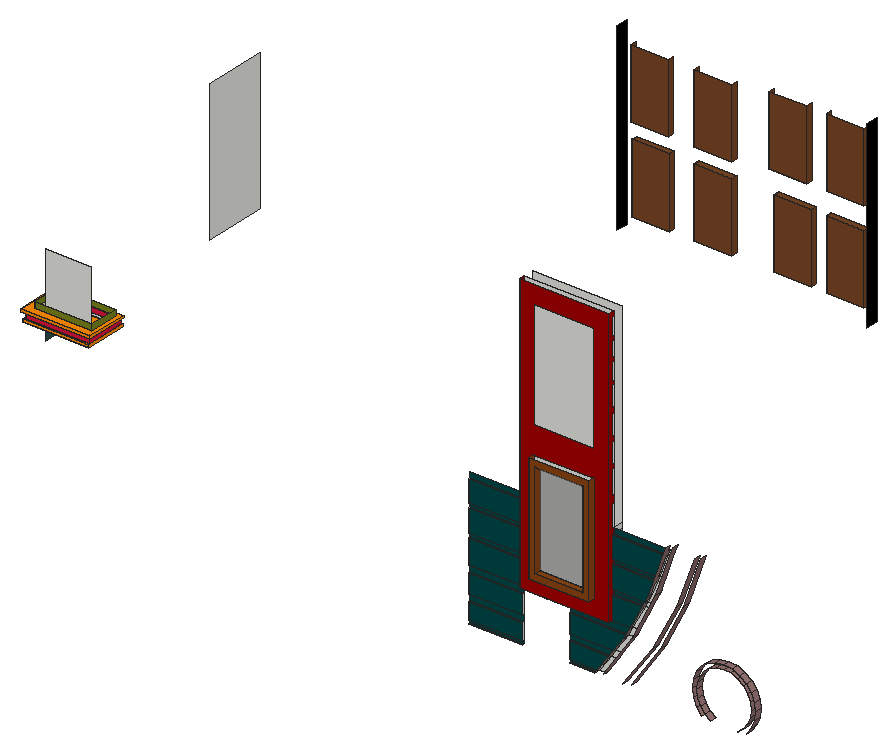
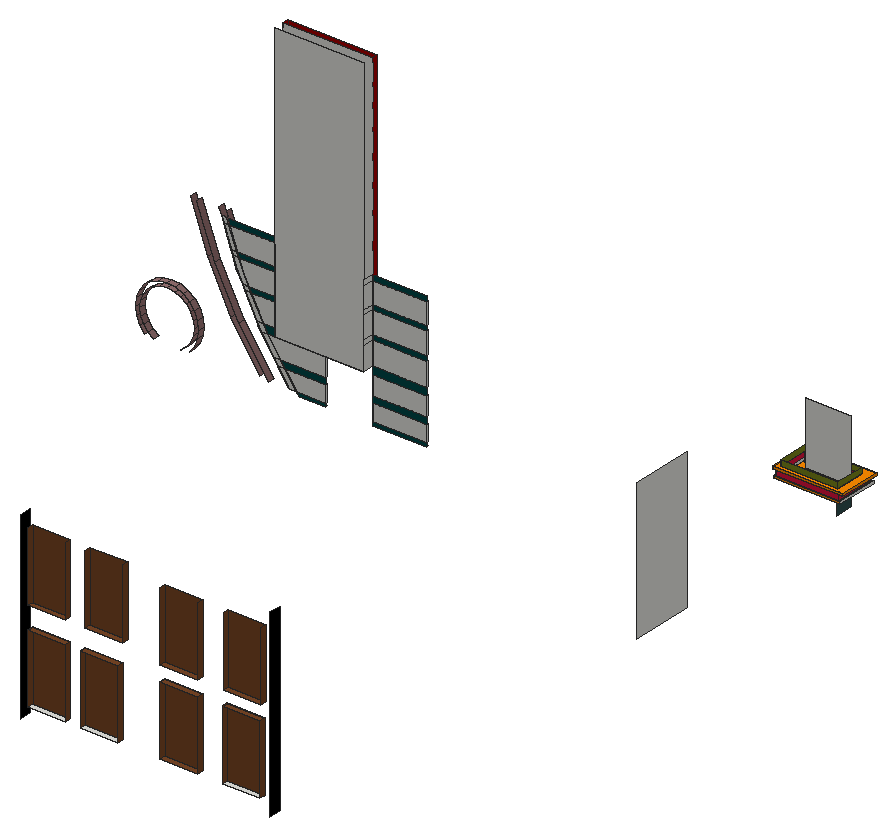
# SketchUp Ruby script. Lengths in inches.
U = 1.inch
M = Sketchup.active_model
def pt(a) = Geom::Point3d.new(a.map { |v| v * U })
def face(e, loops, mat)
  f = e.add_face(loops[0].map { |a| pt(a) })
  loops[1..].each { |l| e.add_face(l.map { |a| pt(a) }).erase! }
  f.material = f.back_material = mat if mat
  f
end
# faces: each face lists its corners as indices into pts; further lists are holes
def faces(e, pts, list, mat = nil) = list.each { |f| face(e, (f[0].is_a?(Array) ? f : [f]).map { |l| l.map { |i| pts[i] } }, mat) }
# xy, xz, yz: faces in a plane at the given z, y or x. An outline is a flat list of corners, or four numbers for a rectangle; further outlines are holes
def ring(l) = l.size == 4 ? [[l[0], l[1]], [l[2], l[1]], [l[2], l[3]], [l[0], l[3]]] : l.each_slice(2).to_a
def flat(e, list, mat, &to3) = list.each { |f| face(e, (f[0].is_a?(Array) ? f : [f]).map { |l| ring(l).map { |u, v| to3.(u, v) } }, mat) }
def xy(e, z, list, mat = nil) = flat(e, list, mat) { |x, y| [x, y, z] }
def xz(e, y, list, mat = nil) = flat(e, list, mat) { |x, z| [x, y, z] }
def yz(e, x, list, mat = nil) = flat(e, list, mat) { |y, z| [x, y, z] }
def lines(e, pts, list) = list.each { |a, b| e.add_line(pt(pts[a]), pt(pts[b])) }
# prism: a flat outline (further loops are holes) pulled along v
def prism(e, loops, v, mat = nil)
  f = face(e, loops, mat); d = Geom::Vector3d.new(v.map { |x| x * U })
  f.pushpull(f.normal.samedirection?(d) ? d.length : -d.length)
end
def box(e, o, s, mat = nil) = prism(e, [[o, [o[0] + s[0], o[1], o[2]], [o[0] + s[0], o[1] + s[1], o[2]], [o[0], o[1] + s[1], o[2]]]], [0, 0, s[2]], mat)
def at(x, y, z, deg = 0) = Geom::Transformation.translation(pt([x, y, z])) * Geom::Transformation.rotation(ORIGIN, Z_AXIS, deg.degrees)
def axes(o, x, y, z) = Geom::Transformation.new([*x, 0, *y, 0, *z, 0, *pt(o).to_a, 1])
def part(name) = M.definitions.add(name)
# library, detail: a bought-in or finely detailed component or shape, given as its bounding box
def library(name, o, s) = part(name).tap { |d| box(d.entities, o, s) }
def detail(e, o, s) = box(e.add_group.entities, o, s)
def put(e, d, t, mat = nil) = e.add_instance(d, t).tap { |i| i.material = mat if mat }
def group(e, t, mat = nil) = e.add_group.tap { |g| g.transformation = t; g.material = mat if mat }.entities
root = M.entities
M.materials.add("[0019_Crimson]").color = [220, 20, 60]
M.materials.add("[0020_Red]").color = [165, 0, 0]
M.materials.add("[0039_DarkOrange]").color = [255, 140, 0]
M.materials.add("[0043_SaddleBrown]").color = [139, 69, 19]
M.materials.add("[0057_DarkKhaki]").color = [122, 132, 27]
M.materials.add("[0078_DarkSlateGray]").color = [47, 79, 79]
M.materials.add("[0119_RosyBrown]").color = [150, 114, 114]
M.materials.add("[0137_Black]").color = [0, 0, 0]
M.materials.add("[Color H08]").color = [0, 71, 71]
M.materials.add("[Translucent Glass Gray]").color = [128, 128, 128]
M.materials["[Translucent Glass Gray]"].alpha = 0.5
M.materials.add("[Wood Veneer 01]").color = [120, 70, 37]
xy(root,126.49,[[221.0625,650.11,247.97,651.11],[271.25,650.11,284.14,651.11]],"[Color H08]")
xy(root,128.2,[[221.0625,650.11,247.97,651.11],[271.25,650.11,285.64,651.11]],"[Color H08]")
xy(root,136.45,[[221.0625,650.11,247.97,651.11],[271.25,650.11,291.42,651.11]],"[Color H08]")
xy(root,139.3125,[[82.93,924.36,101.74,927.36],[153.68,924.36,172.49,927.36],[179.93,924.36,198.74,927.36]])
xy(root,139.3125,[[114.12,924.36,132.93,927.36]],"[Wood Veneer 01]")
xy(root,139.72,[[221.0625,650.11,247.97,651.11],[271.25,650.11,293.72,651.11]],"[Color H08]")
xy(root,149.04,[[221.0625,650.11,247.97,651.11],[271.25,650.11,300.25,651.11]],"[Color H08]")
xy(root,152.96,[[252.74,648.11,252.74,649.11,247.97,649.11,247.97,651.11,271.25,651.11,271.25,649.11,266.58,649.11,266.58,648.11,265.61,648.11,265.61,649.11,253.7,649.11,253.7,648.11],[257.51,648.11,259.2,649.11],[261.76,648.11,263.45,649.11],[247.97,651.11,292.45,656.36]])
xy(root,152.96,[[247.97,648.11,252.74,649.11],[253.7,648.11,257.51,649.11],[259.2,648.11,261.76,649.11],[263.45,648.11,265.61,649.11],[266.58,648.11,266.58,649.11,271.25,649.11,271.25,651.11,292.45,651.11,292.45,648.11]],"[0020_Red]")
xy(root,152.96,[[221.0625,650.11,247.97,651.11],[292.45,650.11,302.3,651.11]],"[Color H08]")
xy(root,160.75,[[255.01,645.11,284.88,648.11]],"[0043_SaddleBrown]")
xy(root,163.75,[[258.01,645.11,281.88,648.11]],"[0043_SaddleBrown]")
xy(root,164.61,[[221.0625,650.11,247.97,651.11],[292.45,650.11,308.39,651.11]],"[Color H08]")
xy(root,166.89,[[221.0625,650.11,247.97,651.11],[292.45,650.11,309.58,651.11]],"[Color H08]")
xy(root,173.8125,[[82.93,924.36,101.74,927.36],[114.12,924.36,132.93,927.36],[153.68,924.36,172.49,927.36],[179.93,924.36,198.74,927.36]],"[Wood Veneer 01]")
xy(root,178.2,[[221.0625,650.11,247.97,651.11],[292.45,650.11,314.52,651.11]],"[Color H08]")
xy(root,180.47,[[221.0625,650.11,247.97,651.11],[292.45,650.11,315.35,651.11]],"[Color H08]")
xy(root,181.25,[[82.37,924.36,101.18,927.36],[114.12,924.36,132.93,927.36]],"[Wood Veneer 01]")
xy(root,184.8125,[[151.49,924.36,170.3,927.36],[179.93,924.36,198.74,927.36]],"[Wood Veneer 01]")
xy(root,185.51,[[7,654.11,29.57,663.11]])
xy(root,185.52,[[2.1875,648.11,33.82,667.68]],"[0039_DarkOrange]")
xy(root,185.54,[[[1.375,647.11,34.38,668.24],[2.1875,648.11,33.82,667.68]]],"[0039_DarkOrange]")
xy(root,186.71,[[33.82,667.68,34.38,668.24]])
xy(root,186.71,[[1.375,647.11,34.38,647.11,34.38,667.68,33.82,667.68,33.82,648.11,2.1875,648.11,2.1875,667.68,33.82,667.68,33.82,668.24,1.375,668.24]],"[0039_DarkOrange]")
xy(root,189.54,[[0,647.11,0,667.68,2.1875,667.68,2.1875,648.11,34.75,648.11,34.75,647.11],[33.82,648.11,33.82,667.68,0,667.68,0,668.24,34.75,668.24,34.75,648.11]],"[0039_DarkOrange]")
xy(root,190.71,[[[0,647.11,34.75,668.24],[4,651.11,32.57,666.11]]],"[0039_DarkOrange]")
xy(root,191.16,[[221.0625,650.11,247.97,651.11],[292.45,650.11,319.27,651.11]],"[Color H08]")
xz(root,645.11,[[[255.01,160.75,284.88,214.75],[258.01,163.75,281.88,211.75]]],"[0043_SaddleBrown]")
xz(root,647.11,[[1.375,185.54,34.38,186.71],[0,189.54,34.75,190.71]],"[0039_DarkOrange]")
xz(root,648.11,[[2.1875,185.52,33.82,185.54],[2.1875,185.54,33.82,186.71]])
xz(root,648.11,[[2.1875,186.71,33.82,189.54]],"[0019_Crimson]")
xz(root,648.11,[[[247.97,152.96,292.45,290.61],[255.01,227.93,284.88,281.93],[255.01,160.75,284.88,214.75]]],"[0020_Red]")
xz(root,648.11,[[258.01,163.75,281.88,211.75]],"[Translucent Glass Gray]")
xz(root,650.11,[[221.0625,128.2,247.97,136.45],[271.25,128.2,285.64,128.2,291.42,136.45,271.25,136.45],[221.0625,139.72,247.97,149.04],[271.25,139.72,293.72,139.72,300.25,149.04,271.25,149.04],[221.0625,152.96,247.97,164.61],
  [292.45,152.96,302.3,152.96,308.39,164.61,292.45,164.61],[221.0625,166.89,247.97,178.2],[292.45,166.89,309.58,166.89,312.23,171.96,314.52,178.2,292.45,178.2],[221.0625,180.47,247.97,191.16],[292.45,180.47,315.35,180.47,319.27,191.16,292.45,191.16]],"[Color H08]")
xz(root,651.11,[[221.0625,128.2,247.97,136.45],[271.25,128.2,271.25,136.45,291.42,136.45,285.64,128.2],[285.64,128.2,289.23,128.2,290.05,129.14,294.98,136.45,291.42,136.45],[291.42,136.45,294.98,136.45,297.18,139.72,293.72,139.72],[221.0625,139.72,247.97,149.04],
  [271.25,139.72,271.25,149.04,300.25,149.04,293.72,139.72],[293.72,139.72,297.18,139.72,303.45,149.04,300.25,149.04],[300.25,149.04,303.45,149.04,304.36,150.39,305.64,152.96,302.3,152.96],[221.0625,152.96,247.97,164.61],[247.97,152.96,292.45,290.61],
  [292.45,152.96,292.45,164.61,308.39,164.61,302.3,152.96],[302.3,152.96,305.64,152.96,311.48,164.61,308.39,164.61],[308.39,164.61,311.48,164.61,312.62,166.89,309.58,166.89],[221.0625,166.89,247.97,178.2],[292.45,166.89,292.45,178.2,314.52,178.2,312.23,171.96,309.58,166.89],
  [309.58,166.89,312.62,166.89,315.82,173.3,317.53,178.2,314.52,178.2,312.23,171.96],[314.52,178.2,317.53,178.2,318.32,180.47,315.35,180.47],[221.0625,180.47,247.97,191.16],[292.45,180.47,292.45,191.16,319.27,191.16,315.35,180.47],[315.35,180.47,318.32,180.47,322.05,191.16,319.27,191.16],
  [319.27,191.16,322.05,191.16,323.04,194,320.32,194]])
xz(root,651.11,[[4,190.71,32.57,193.52]],"[0057_DarkKhaki]")
xz(root,651.11,[[221.0625,126.49,247.97,128.2],[271.25,126.49,284.14,126.49,285.39,127.86,285.64,128.2,271.25,128.2],[221.0625,136.45,247.97,139.72],[271.25,136.45,291.42,136.45,293.72,139.72,271.25,139.72],[221.0625,149.04,247.97,152.96],
  [271.25,149.04,300.25,149.04,302.3,152.96,271.25,152.96],[221.0625,164.61,247.97,166.89],[292.45,164.61,308.39,164.61,309.58,166.89,292.45,166.89],[221.0625,178.2,247.97,180.47],[292.45,178.2,314.52,178.2,315.35,180.47,292.45,180.47],
  [221.0625,191.16,247.97,194],[292.45,191.16,319.27,191.16,320.32,194,292.45,194]],"[Color H08]")
xz(root,654.11,[[7,185.51,29.57,216.77]])
xz(root,656.36,[[247.97,152.96,292.45,290.61]])
xz(root,666.11,[[4,190.71,32.57,193.52]],"[0057_DarkKhaki]")
xz(root,667.68,[[2.1875,185.52,33.82,185.54],[2.1875,185.54,33.82,186.71]])
xz(root,667.68,[[2.1875,186.71,33.82,189.54]],"[0019_Crimson]")
xz(root,668.24,[[1.375,185.54,34.38,186.71],[0,189.54,34.75,190.71]],"[0039_DarkOrange]")
xz(root,924.36,[[82.93,139.3125,101.74,173.8125],[114.12,139.3125,132.93,173.8125],[153.68,139.3125,172.49,173.8125],[179.93,139.3125,198.74,173.8125],[82.37,181.25,101.18,215.75],
  [114.12,181.25,132.93,215.75],[151.49,184.8125,170.3,219.3125],[179.93,184.8125,198.74,219.3125]],"[Wood Veneer 01]")
yz(root,0,[[647.11,189.54,668.24,190.71]],"[0039_DarkOrange]")
yz(root,1.375,[[647.11,185.54,668.24,186.71]])
yz(root,2.1875,[[648.11,185.52,667.68,185.54],[648.11,185.54,667.68,186.71]])
yz(root,2.1875,[[648.11,186.71,667.68,189.54]],"[0019_Crimson]")
yz(root,4,[[651.11,185.51,666.11,185.52],[651.11,185.52,666.11,190.71]])
yz(root,4,[[651.11,190.71,666.11,193.52]],"[0057_DarkKhaki]")
yz(root,7,[[756.4375,176,787.78,245.51]])
yz(root,7,[[654.11,176,663.11,185.51]],"[0078_DarkSlateGray]")
yz(root,32.57,[[651.11,190.71,666.11,193.52]],"[0057_DarkKhaki]")
yz(root,33.82,[[648.11,185.52,667.68,185.54],[648.11,185.54,667.68,186.71]])
yz(root,33.82,[[648.11,186.71,667.68,189.54]],"[0019_Crimson]")
yz(root,34.38,[[647.11,185.54,668.24,186.71]],"[0039_DarkOrange]")
yz(root,34.75,[[647.11,189.54,668.24,190.71]],"[0039_DarkOrange]")
yz(root,78.125,[[921.36,132.83,927.36,224.07]],"[0137_Black]")
yz(root,82.37,[[924.36,181.25,927.36,215.75]],"[Wood Veneer 01]")
yz(root,82.93,[[924.36,139.3125,927.36,173.8125]],"[Wood Veneer 01]")
yz(root,101.18,[[924.36,181.25,927.36,215.75]],"[Wood Veneer 01]")
yz(root,101.74,[[924.36,139.3125,927.36,173.8125]],"[Wood Veneer 01]")
yz(root,114.12,[[924.36,139.3125,927.36,173.8125],[924.36,181.25,927.36,215.75]],"[Wood Veneer 01]")
yz(root,132.93,[[924.36,139.3125,927.36,173.8125],[924.36,181.25,927.36,215.75]],"[Wood Veneer 01]")
yz(root,151.49,[[924.36,184.8125,927.36,219.3125]],"[Wood Veneer 01]")
yz(root,153.68,[[924.36,139.3125,927.36,173.8125]],"[Wood Veneer 01]")
yz(root,170.3,[[924.36,184.8125,927.36,219.3125]],"[Wood Veneer 01]")
yz(root,172.49,[[924.36,139.3125,927.36,173.8125]],"[Wood Veneer 01]")
yz(root,179.93,[[924.36,139.3125,927.36,173.8125],[924.36,184.8125,927.36,219.3125]],"[Wood Veneer 01]")
yz(root,198.74,[[924.36,139.3125,927.36,173.8125],[924.36,184.8125,927.36,219.3125]],"[Wood Veneer 01]")
yz(root,202.43,[[921.36,132.83,927.36,224.07]],"[0137_Black]")
yz(root,221.0625,[[650.11,128.2,651.11,136.45],[650.11,139.72,651.11,149.04],[650.11,152.96,651.11,164.61],[650.11,166.89,651.11,178.2],[650.11,180.47,651.11,191.16]])
yz(root,247.97,[[650.11,128.2,651.11,136.45],[650.11,139.72,651.11,149.04],[650.11,152.96,651.11,164.61],[651.11,152.96,656.36,164.61],[651.11,164.61,656.36,166.89],
  [650.11,166.89,651.11,178.2],[651.11,166.89,656.36,178.2],[651.11,178.2,656.36,180.47],[650.11,180.47,651.11,191.16],[651.11,180.47,656.36,191.16],
  [651.11,191.16,656.36,194]])
yz(root,247.97,[[648.11,152.96,648.11,290.61,651.11,290.61,651.11,288.67,650.11,288.67,650.11,279.73,651.11,279.73,651.11,278.01,650.11,278.01,650.11,270.44,651.11,270.44,651.11,268.56,650.11,268.56,650.11,259.56,651.11,259.56,651.11,258.11,650.11,258.11,650.11,247.73,651.11,247.73,651.11,245.03,650.11,245.03,650.11,234.84,651.11,234.84,651.11,232.54,650.11,232.54,650.11,222.41,651.11,222.41,651.11,220.65,650.11,220.65,650.11,208.59,651.11,208.59,651.11,204.94,650.11,204.94,650.11,194,651.11,194,651.11,191.16,650.11,191.16,650.11,180.47,651.11,180.47,651.11,178.2,650.11,178.2,650.11,166.89,651.11,166.89,651.11,164.61,650.11,164.61,650.11,152.96]],"[0020_Red]")
yz(root,255.01,[[645.11,160.75,648.11,214.75]],"[0043_SaddleBrown]")
yz(root,258.01,[[645.11,163.75,648.11,211.75]],"[0043_SaddleBrown]")
yz(root,271.25,[[650.11,128.2,651.11,136.45],[650.11,139.72,651.11,149.04]])
yz(root,281.88,[[645.11,163.75,648.11,211.75]],"[0043_SaddleBrown]")
yz(root,284.88,[[645.11,160.75,648.11,214.75]],"[0043_SaddleBrown]")
yz(root,292.45,[[650.11,152.96,651.11,164.61],[651.11,152.96,656.36,164.61],[651.11,164.61,656.36,166.89],[650.11,166.89,651.11,178.2],[651.11,166.89,656.36,178.2],
  [651.11,178.2,656.36,180.47],[650.11,180.47,651.11,191.16],[651.11,180.47,656.36,191.16],[651.11,191.16,656.36,194]])
yz(root,292.45,[[648.11,152.96,650.11,152.96,650.11,164.61,651.11,164.61,651.11,166.89,650.11,166.89,650.11,178.2,651.11,178.2,651.11,180.47,650.11,180.47,650.11,191.16,651.11,191.16,651.11,194,650.11,194,650.11,204.94,651.11,204.94,651.11,208.59,650.11,208.59,650.11,220.65,651.11,220.65,651.11,222.41,650.11,222.41,650.11,232.54,651.11,232.54,651.11,234.84,650.11,234.84,650.11,245.03,651.11,245.03,651.11,247.73,650.11,247.73,650.11,258.11,651.11,258.11,651.11,259.56,650.11,259.56,650.11,268.56,651.11,268.56,651.11,270.44,650.11,270.44,650.11,278.01,651.11,278.01,651.11,279.73,650.11,279.73,650.11,288.67,651.11,288.67,651.11,290.61,648.11,290.61]],"[0020_Red]")
p = [[343.3125,651.11,126.95],[340.5,651.11,129.1],[340.5,648.11,129.1],[343.3125,648.11,126.95],[359.66,651.11,129.1],[356.86,651.11,126.95],
  [356.86,648.11,126.95],[359.66,648.11,129.1],[336.39,651.11,130.78],[338.9,651.11,127.5],[338.9,648.11,127.5],[336.39,648.11,130.78],
  [361.27,651.11,127.5],[363.78,651.11,130.78],[363.78,648.11,130.78],[361.27,648.11,127.5],[285.64,651.11,128.2],[285.39,651.11,127.86],
  [285.39,648.11,127.86],[300.25,648.11,149.04],[300.25,650.11,149.04],[293.72,650.11,139.72],[293.72,651.11,139.72],[291.42,651.11,136.45],
  [291.42,650.11,136.45],[285.64,650.11,128.2],[314.33,651.11,149.04],[299.47,651.11,127.86],[299.47,648.11,127.86],[314.33,648.11,149.04],
  [290.05,651.11,129.14],[294.98,651.11,136.45],[297.18,651.11,139.72],[303.45,651.11,149.04],[304.36,651.11,150.39],[304.36,648.11,150.39],
  [290.05,648.11,129.14],[304.13,651.11,129.14],[318.4375,651.11,150.39],[318.4375,648.11,150.39],[304.13,648.11,129.14],[338.35,651.11,131.91],
  [338.35,648.11,131.91],[361.82,651.11,131.91],[361.82,648.11,131.91],[334.8125,651.11,134.59],[334.8125,648.11,134.59],[365.36,651.11,134.59],
  [365.36,648.11,134.59],[337,651.11,135.18],[337,648.11,135.18],[363.17,651.11,135.18],[363.17,648.11,135.18],[334.27,651.11,138.68],
  [334.27,648.11,138.68],[365.9,651.11,138.68],[365.9,648.11,138.68],[336.54,651.11,138.68],[336.54,648.11,138.68],[363.63,651.11,138.68],
  [363.63,648.11,138.68],[334.8125,651.11,142.77],[334.8125,648.11,142.77],[337,651.11,142.1875],[337,648.11,142.1875],[363.17,651.11,142.1875],
  [363.17,648.11,142.1875],[365.36,651.11,142.77],[365.36,648.11,142.77],[300.25,651.11,149.04],[338.35,651.11,145.46],[338.35,648.11,145.46],
  [361.82,651.11,145.46],[361.82,648.11,145.46],[336.39,651.11,146.59],[336.39,648.11,146.59],[363.78,651.11,146.59],[363.78,648.11,146.59],
  [340.5,651.11,148.26],[340.5,648.11,148.26],[359.66,651.11,148.26],[359.66,648.11,148.26],[338.9,651.11,149.86],[338.9,648.11,149.86],
  [361.27,651.11,149.86],[361.27,648.11,149.86],[343.3125,651.11,150.41],[343.3125,648.11,150.41],[356.86,651.11,150.41],[356.86,648.11,150.41],
  [302.3,651.11,152.96],[312.23,648.11,171.96],[312.23,650.11,171.96],[309.58,650.11,166.89],[309.58,651.11,166.89],[308.39,651.11,164.61],
  [308.39,650.11,164.61],[302.3,650.11,152.96],[326.31,651.11,171.96],[326.31,648.11,171.96],[342.18,651.11,152.375],[342.18,648.11,152.375],
  [357.99,651.11,152.375],[357.99,648.11,152.375],[305.64,651.11,152.96],[311.48,651.11,164.61],[312.62,651.11,166.89],[315.82,651.11,173.3],
  [315.82,648.11,173.3],[329.9,651.11,173.3],[329.9,648.11,173.3],[346.58,651.11,151.77],[346.58,648.11,151.77],[353.59,651.11,151.77],
  [353.59,648.11,151.77],[350.08,651.11,152.23],[350.08,648.11,152.23],[345.99,651.11,153.96],[345.99,648.11,153.96],[354.18,651.11,153.96],
  [354.18,648.11,153.96],[350.08,651.11,154.49],[350.08,648.11,154.49],[312.23,651.11,171.96],[315.35,651.11,180.47],[314.52,651.11,178.2],
  [314.52,650.11,178.2],[321.14,648.11,196.24],[321.14,650.11,196.24],[320.32,650.11,194],[320.32,651.11,194],[319.27,651.11,191.16],
  [319.27,650.11,191.16],[315.35,650.11,180.47],[335.22,651.11,196.24],[335.22,648.11,196.24],[317.53,651.11,178.2],[318.32,651.11,180.47],
  [322.05,651.11,191.16],[323.04,651.11,194],[324.26,651.11,197.49],[324.26,648.11,197.49],[338.33,651.11,197.49],[338.33,648.11,197.49],
  [32.57,651.11,190.71],[32.57,651.11,185.51],[2.1875,667.68,190.71],[2.1875,667.68,189.54],[33.82,648.11,189.54],[33.82,648.11,190.71],
  [33.82,667.68,189.54],[33.82,667.68,190.71],[32.57,666.11,185.51],[32.57,666.11,190.71]]
faces(root,p,[[0,1,2,3],[4,5,6,7],[8,9,10,11],[12,13,14,15],[16,17,18,19,20,21,22,23,24,25],[26,27,28,29],[30,31,32,33,34,35,36],[37,38,39,40],
  [1,41,42,2],[43,4,7,44],[45,8,11,46],[13,47,48,14],[41,49,50,42],[51,43,44,52],[53,45,46,54],[47,55,56,48],
  [49,57,58,50],[59,51,52,60],[61,53,54,62],[57,63,64,58],[65,59,60,66],[55,67,68,56],[63,70,71,64],[72,65,66,73],
  [74,61,62,75],[67,76,77,68],[70,78,79,71],[80,72,73,81],[82,74,75,83],[76,84,85,77],[78,86,87,79],[88,80,81,89],
  [90,69,20,19,91,92,93,94,95,96,97],[98,26,29,99],[100,82,83,101],[84,102,103,85],[34,104,105,106,107,108,35],[38,109,110,39],[86,111,112,87],[113,88,89,114],
  [111,115,116,112],[115,113,114,116],[117,100,101,118],[102,119,120,103],[121,117,118,122],[119,121,122,120],[124,125,126,92,91,127,128,129,130,131,132,133],[134,98,99,135],
  [107,136,137,138,139,140,141,108],[109,142,143,110]],"[0119_RosyBrown]")
faces(root,p,[[23,16,25,24],[69,22,21,20],[95,90,97,96],[123,94,93,92],[125,123,92,126],[131,124,133,132]])
lines(root,p,[[144,145],[146,147],[148,149],[150,151],[152,153]])
